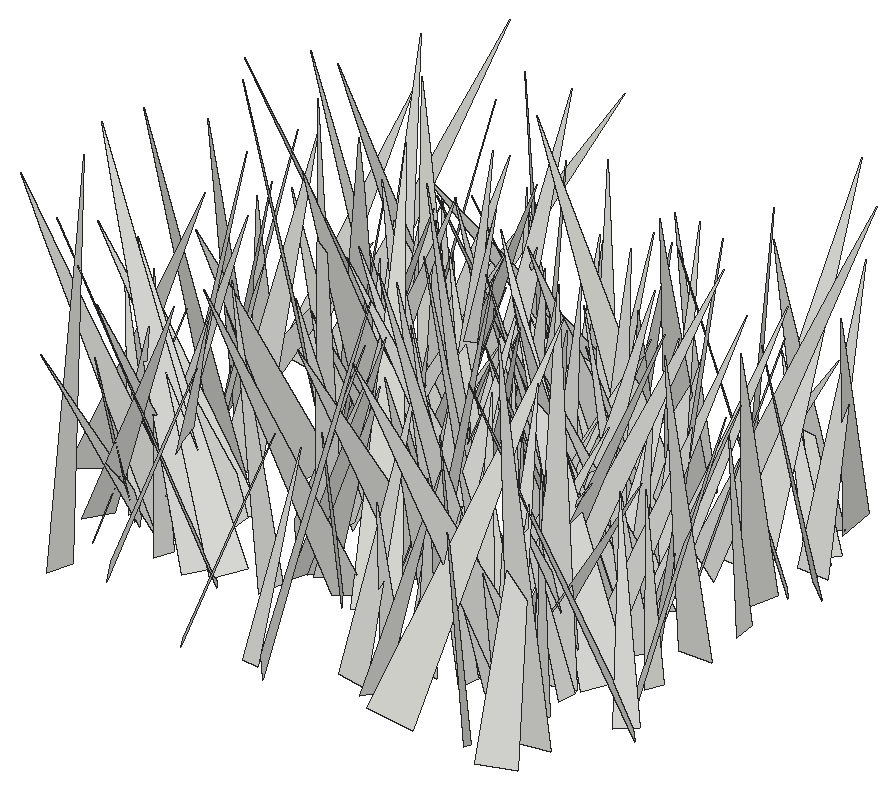
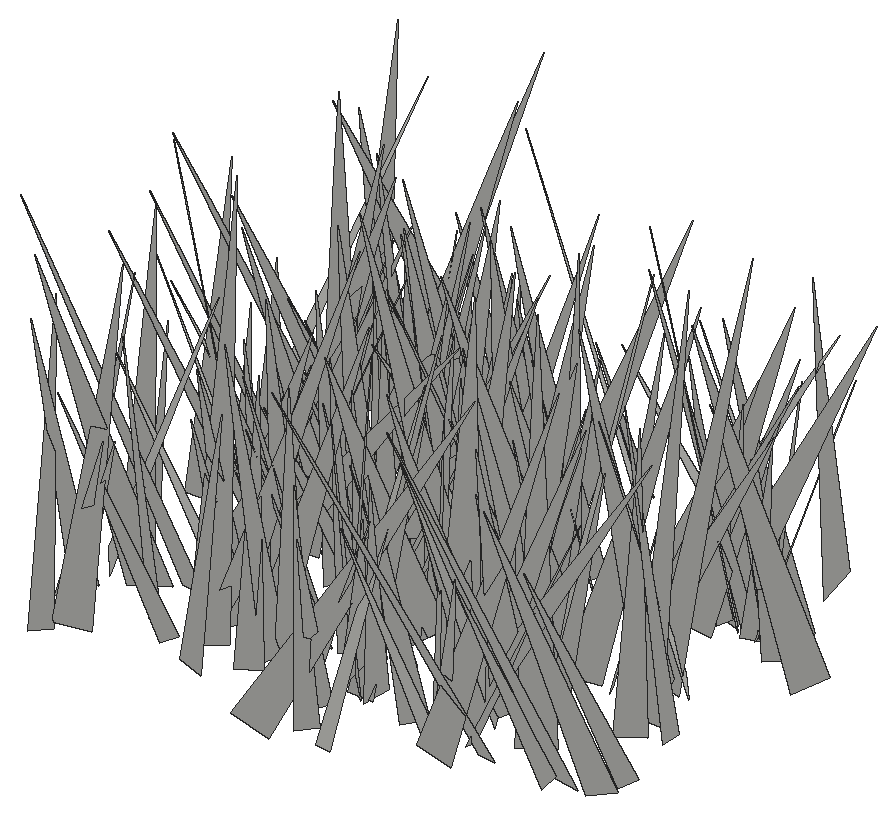
# SketchUp Ruby script. Lengths in inches.
U = 1.inch
M = Sketchup.active_model
def pt(a) = Geom::Point3d.new(a.map { |v| v * U })
def face(e, loops, mat)
  f = e.add_face(loops[0].map { |a| pt(a) })
  loops[1..].each { |l| e.add_face(l.map { |a| pt(a) }).erase! }
  f.material = f.back_material = mat if mat
  f
end
# faces: each face lists its corners as indices into pts; further lists are holes
def faces(e, pts, list, mat = nil) = list.each { |f| face(e, (f[0].is_a?(Array) ? f : [f]).map { |l| l.map { |i| pts[i] } }, mat) }
# xy, xz, yz: faces in a plane at the given z, y or x. An outline is a flat list of corners, or four numbers for a rectangle; further outlines are holes
def ring(l) = l.size == 4 ? [[l[0], l[1]], [l[2], l[1]], [l[2], l[3]], [l[0], l[3]]] : l.each_slice(2).to_a
def flat(e, list, mat, &to3) = list.each { |f| face(e, (f[0].is_a?(Array) ? f : [f]).map { |l| ring(l).map { |u, v| to3.(u, v) } }, mat) }
def xy(e, z, list, mat = nil) = flat(e, list, mat) { |x, y| [x, y, z] }
def xz(e, y, list, mat = nil) = flat(e, list, mat) { |x, z| [x, y, z] }
def yz(e, x, list, mat = nil) = flat(e, list, mat) { |y, z| [x, y, z] }
def lines(e, pts, list) = list.each { |a, b| e.add_line(pt(pts[a]), pt(pts[b])) }
# prism: a flat outline (further loops are holes) pulled along v
def prism(e, loops, v, mat = nil)
  f = face(e, loops, mat); d = Geom::Vector3d.new(v.map { |x| x * U })
  f.pushpull(f.normal.samedirection?(d) ? d.length : -d.length)
end
def box(e, o, s, mat = nil) = prism(e, [[o, [o[0] + s[0], o[1], o[2]], [o[0] + s[0], o[1] + s[1], o[2]], [o[0], o[1] + s[1], o[2]]]], [0, 0, s[2]], mat)
def at(x, y, z, deg = 0) = Geom::Transformation.translation(pt([x, y, z])) * Geom::Transformation.rotation(ORIGIN, Z_AXIS, deg.degrees)
def axes(o, x, y, z) = Geom::Transformation.new([*x, 0, *y, 0, *z, 0, *pt(o).to_a, 1])
def part(name) = M.definitions.add(name)
# library, detail: a bought-in or finely detailed component or shape, given as its bounding box
def library(name, o, s) = part(name).tap { |d| box(d.entities, o, s) }
def detail(e, o, s) = box(e.add_group.entities, o, s)
def put(e, d, t, mat = nil) = e.add_instance(d, t).tap { |i| i.material = mat if mat }
def group(e, t, mat = nil) = e.add_group.tap { |g| g.transformation = t; g.material = mat if mat }.entities
root = M.entities
c1 = part("fur_instance\#9")
p = [[0.8125,0,1.79],[0.67,-0.02,1.48],[0,-0.11,0],[0,0.11,0]]
faces(c1.entities,p,[[0,1,2,3]])
put(root,c1,axes([118.52,285.79,-27.1],[3.43862,2.40363,0.16823],[2.31203,-3.37399,0.94893],[-0.67841,0.6845,4.08669]))
put(root,c1,axes([121.77,286.14,-27.1],[5.53821,4.98185,1.27941],[5.04776,-5.62536,0.05401],[-0.98782,-0.81487,7.449]))
put(root,c1,axes([125.91,287.1,-27.1],[4.66394,-1.20705,1.00362],[-1.36601,-4.67089,0.73033],[-0.77347,0.97077,4.76192]))
put(root,c1,axes([132.45,287.6,-27.1],[0.36283,-7.33481,3.26148],[-7.98321,-0.67122,-0.62142],[-0.83968,3.21222,7.31744]))
put(root,c1,axes([132.47,285.72,-27.1],[-2.78795,6.31949,0.96814],[6.36227,2.84625,-0.25738],[0.62828,-0.78026,6.90234]))
put(root,c1,axes([121.28,286.12,-27.1],[1.03899,3.82207,0.22987],[3.79032,-1.06041,0.49963],[-0.54276,-0.08876,3.92914]))
put(root,c1,axes([131.54,287.22,-27.1],[2.89571,-2.97183,2.13904],[-3.49598,-3.05481,0.48854],[-1.08874,1.90494,4.12046]))
put(root,c1,axes([130.74,286.27,-27.1],[-5.03149,-1.83162,1.20846],[-2.18082,4.50919,-2.24552],[0.24343,2.5384,4.86091]))
put(root,c1,axes([129.28,291.125,-27.1],[-7.73279,0.49202,2.83462],[1.75633,7.24586,3.53356],[2.27869,-3.91518,6.89581]))
put(root,c1,axes([125.46,288.78,-27.1],[2.03457,-2.99845,1.01926],[-3.06758,-2.16697,-0.25148],[-0.78708,0.69471,3.61482]))
put(root,c1,axes([113.4,288.13,-27.1],[4.3525,2.53578,0.43229],[2.57081,-4.2585,-0.90411],[0.08934,-0.99816,4.9555]))
put(root,c1,axes([124.8,287.36,-27.1],[0.44242,5.64748,1.29703],[5.78226,-0.34572,-0.46699],[0.37666,-1.32609,5.6455]))
put(root,c1,axes([127.49,286.0625,-27.1],[-1.94232,7.80928,1.11049],[7.41359,2.19794,-2.48968],[2.69386,-0.41817,7.65238]))
put(root,c1,axes([134.57,290.7,-27.1],[-5.605,-5.08718,0.25266],[-5.09303,5.60246,-0.18084],[0.06544,0.30374,7.56721]))
put(root,c1,axes([111.93,287.25,-27.1],[-7.13651,-0.0123,2.39844],[-0.61978,7.28244,-1.80677],[2.31701,1.91008,6.90402]))
put(root,c1,axes([126.49,289.33,-27.1],[0.16475,-3.83195,1.51207],[-4.1166,-0.0965,0.20397],[0.15418,1.51796,3.83006]))
put(root,c1,axes([126.33,289.23,-27.1],[2.59266,-2.6088,0.97622],[-2.78019,-2.50569,0.68761],[-0.17141,1.18171,3.61316]))
put(root,c1,axes([129.45,289.94,-27.1],[-0.93338,-7.69941,2.7531],[-7.87622,0.10215,-2.38461],[-2.19672,2.90522,7.38009]))
put(root,c1,axes([111.72,291.98,-27.1],[-3.93384,-2.91751,0.42121],[-2.51987,3.69278,2.04402],[1.52955,-1.41982,4.45073]))
put(root,c1,axes([116.91,289.72,-27.1],[-5.49378,-4.48735,0.1731],[-4.21573,5.05933,-2.64174],[-1.54724,2.14821,6.58325]))
put(root,c1,axes([120.97,292.02,-27.1],[0.32689,-6.93131,1.01824],[-6.72809,-0.59471,-1.88835],[-1.95261,0.88881,6.67713]))
put(root,c1,axes([111.3,291.95,-27.1],[-2.16154,-4.08693,0.6496],[-3.73051,2.24163,1.68984],[1.79115,-0.26331,4.30345]))
put(root,c1,axes([110.67,290.95,-27.1],[5.28357,-2.5058,0.04843],[-2.504,-5.27298,0.35108],[0.10676,0.33794,5.83712]))
put(root,c1,axes([120.83,291.77,-27.1],[-2.98653,-2.99705,1.42564],[-2.58075,3.30304,1.53746],[2.08674,-0.20437,3.94181]))
put(root,c1,axes([128.03,289.86,-27.1],[-6.43885,-0.2283,0.73687],[-0.34147,6.39798,-1.00159],[0.69173,1.03328,6.36457]))
put(root,c1,axes([113.85,291.4,-27.1],[-2.36054,6.29762,2.85628],[6.53149,1.03928,3.10644],[-2.27111,-3.55673,5.96508]))
put(root,c1,axes([113.81,292.71,-27.1],[0.77993,-5.26102,0.56712],[-5.12867,-0.89269,-1.22806],[-1.30258,0.36472,5.1748]))
put(root,c1,axes([111.5,289.76,-27.1],[4.04394,2.43918,0.42992],[2.39305,-4.06014,0.52577],[-0.63852,0.23141,4.69325]))
put(root,c1,axes([131.56,289.47,-27.1],[-4.31752,-0.25034,0.73123],[-0.52227,4.00392,-1.71296],[0.56974,1.77322,3.97108]))
put(root,c1,axes([131.33,291.0625,-27.1],[-3.91396,0.19988,0.40503],[0.19284,3.93443,-0.07818],[0.40843,0.05784,3.91828]))
put(root,c1,axes([113.33,291.49,-27.1],[4.73571,-1.08461,0.9225],[-1.0987,-4.82145,-0.02851],[-0.90568,0.17765,4.85824]))
put(root,c1,axes([118.53,290.67,-27.1],[-5.56537,0.35389,1.01892],[0.25962,5.63719,-0.53984],[1.04691,0.48332,5.55042]))
put(root,c1,axes([126.13,289.2,-27.1],[6.62272,2.03005,2.53711],[1.31072,-6.93962,2.13125],[-2.97322,1.46257,6.59085]))
put(root,c1,axes([130.98,293.18,-27.1],[-4.32918,-1.79601,0.73607],[-1.48596,4.22424,1.56749],[1.24875,-1.19977,4.41706]))
put(root,c1,axes([114.15,290.24,-27.1],[-5.02502,0.15502,0.9974],[-0.08895,4.97687,-1.22169],[1.00545,1.21508,4.87671]))
put(root,c1,axes([128.1,290.34,-27.1],[-0.91047,5.0165,1.03079],[5.11456,0.83694,0.44447],[-0.2628,-1.09133,5.07905]))
put(root,c1,axes([116.74,290.58,-27.1],[-3.94655,4.7323,0.06828],[4.56087,3.77904,1.70056],[-1.26405,-1.13963,5.92267]))
put(root,c1,axes([118.87,292.26,-27.1],[6.16535,-1.94029,0.16764],[-1.94054,-6.16752,-0.01601],[-0.16472,0.03505,6.46343]))
put(root,c1,axes([134.27,290.66,-27.1],[-2.51117,3.39602,0.58609],[3.43959,2.51478,0.1658],[0.21361,-0.57041,4.22035]))
put(root,c1,axes([115.94,290.33,-27.1],[-4.22364,6.9226,0.63988],[6.72709,3.88063,2.42031],[-1.75445,-1.78585,7.73974]))
put(root,c1,axes([121.8,295.03,-27.1],[6.11084,-2.63091,1.80363],[-1.49433,-5.80472,-3.40432],[-2.81811,-2.62692,5.71618]))
put(root,c1,axes([110.3,292.7,-27.1],[2.04033,-4.0488,0.48109],[-4.03745,-1.93127,0.8697],[0.56854,0.81522,4.44965]))
put(root,c1,axes([130.5,291.42,-27.1],[1.64686,-6.77743,3.62945],[-7.62252,-1.92308,-0.13234],[-1.0018,3.49096,6.97339]))
put(root,c1,axes([119.25,292.66,-27.1],[4.36325,-2.68491,0.18726],[-2.69098,-4.34538,0.39756],[0.04948,0.43666,5.1077]))
put(root,c1,axes([112.15,291.73,-27.1],[3.4737,5.90005,1.74495],[6.11319,-3.08303,-1.74525],[0.69596,-2.36778,6.62052]))
put(root,c1,axes([128.96,291.46,-27.1],[4.72114,-1.50275,0.05764],[-1.46013,-4.53503,1.361],[0.36002,1.31378,4.76394]))
put(root,c1,axes([113.13,291.31,-27.1],[5.7382,5.20942,1.87337],[5.41352,-5.84467,-0.3291],[-1.15821,-1.50876,7.74318]))
put(root,c1,axes([111.57,291.66,-27.1],[-2.88957,-1.62735,2.00469],[-2.2228,3.09866,-0.68855],[1.31385,1.66334,3.24403]))
put(root,c1,axes([128.09,293.5625,-27.1],[4.34491,0.59069,1.09524],[0.90101,-4.23706,-1.28924],[-0.85828,-1.45776,4.19106]))
put(root,c1,axes([111.79,292.02,-27.1],[-2.18486,3.79279,1.02862],[3.92891,2.13324,0.47945],[0.08359,-1.13179,4.35074]))
put(root,c1,axes([122.86,294.39,-27.1],[2.86729,-4.50295,0.62999],[-4.43501,-2.93396,-0.78577],[-1.00209,0.10064,5.2802]))
put(root,c1,axes([124.1,293.9375,-27.1],[1.75802,-6.33898,1.96931],[-6.51413,-2.03906,-0.74828],[-1.27556,1.67662,6.53555]))
put(root,c1,axes([114.79,293.84,-27.1],[-6.1435,0.43905,0.01492],[0.43419,6.03663,1.1429],[-0.06685,-1.14104,6.05221]))
put(root,c1,axes([125.51,290.25,-27.1],[-5.11664,3.91829,0.85035],[3.38571,4.96082,-2.48663],[2.14782,1.51438,5.94556]))
put(root,c1,axes([127.67,291.82,-27.1],[-6.96753,-1.64469,0.65915],[-1.76863,6.61713,-2.18437],[0.10697,2.27915,6.81763]))
put(root,c1,axes([127.39,293.35,-27.1],[4.14484,0.5886,1.74948],[0.68446,-4.48393,-0.11303],[-1.71425,-0.36717,4.1849]))
put(root,c1,axes([108.24,293.32,-27.1],[6.2285,-2.9564,0.62521],[-3.02175,-6.08711,1.31964],[0.01382,1.46019,6.76705]))
put(root,c1,axes([130.64,294.27,-27.1],[-3.35511,-5.27651,0.83113],[-5.27558,3.11951,-1.49198],[-0.83701,1.48869,6.07225]))
put(root,c1,axes([123.48,295.4375,-27.1],[7.4678,0.08394,0.57516],[0.2355,-7.21321,-2.00499],[-0.53141,-2.01703,7.1941]))
put(root,c1,axes([131.8125,292.59,-27.1],[-7.18183,4.15456,0.03319],[4.14203,7.15453,0.70461],[-0.3242,-0.62648,8.26695]))
put(root,c1,axes([125.59,294.01,-27.1],[2.92691,3.10527,0.26779],[2.82947,-2.4932,-2.01476],[1.3071,-1.55642,3.76168]))
put(root,c1,axes([133.22,293.55,-27.1],[3.01506,-0.72225,2.0256],[-1.00024,-3.559,0.21985],[-1.90373,0.72607,3.09256]))
put(root,c1,axes([114.72,293.96,-27.1],[-4.43376,3.47486,0.22998],[3.34427,4.14468,1.85019],[-0.97128,-1.59146,5.32068]))
put(root,c1,axes([126.64,293.03,-27.1],[0.2906,4.64928,0.9365],[4.41539,0.07727,-1.75374],[1.73123,-0.9775,4.31562]))
put(root,c1,axes([116.67,294.36,-27.1],[3.8282,2.91024,0.83789],[3.01788,-3.55309,-1.44728],[0.25298,-1.65308,4.58585]))
put(root,c1,axes([119.48,292.55,-27.1],[4.39596,-0.31282,2.17467],[-1.10489,-4.51925,1.5834],[-1.89902,1.90528,4.11281]))
put(root,c1,axes([128.0625,292.4,-27.1],[6.72656,-0.08852,1.07497],[-0.40385,-6.50233,1.99163],[-1.00015,2.03024,6.42556]))
put(root,c1,axes([122.38,291.72,-27.1],[-3.14428,7.71271,0.49149],[7.72648,3.12546,0.38342],[-0.17032,-0.59964,8.32018]))
put(root,c1,axes([123.1,291.56,-27.1],[4.98815,3.01806,0.37753],[2.59556,-4.60182,2.49383],[-1.58564,1.9615,5.26983]))
put(root,c1,axes([112.21,296.47,-27.1],[-2.39726,-7.68863,1.50052],[-7.81274,2.46126,0.12966],[0.5725,1.39306,8.05265]))
put(root,c1,axes([128.03,296.89,-27.1],[0.49777,-7.47829,0.86543],[-7.52286,-0.52678,-0.22508],[-0.28353,0.84808,7.49146]))
put(root,c1,axes([126.61,293.875,-27.1],[-4.17339,1.81444,1.20525],[1.74242,4.34394,-0.50613],[1.30721,0.0026,4.52253]))
put(root,c1,axes([125.91,293.68,-27.1],[-7.81157,-0.92448,1.21309],[-1.13809,7.74743,-1.42443],[1.01538,1.5715,7.73604]))
put(root,c1,axes([117.86,296.0625,-27.1],[-4.50462,1.14541,2.32905],[1.86637,4.67145,1.31236],[1.80364,-1.97324,4.45884]))
put(root,c1,axes([133.42,292.21,-27.1],[3.56764,3.88458,0.34534],[3.52617,-3.41301,1.96335],[-1.66594,1.09483,4.89523]))
put(root,c1,axes([124.53,296.16,-27.1],[-6.85321,0.30824,0.48855],[0.41589,6.6696,1.62593],[0.40091,-1.64973,6.66467]))
put(root,c1,axes([114.72,297.91,-27.1],[4.75153,-4.99406,0.9078],[-4.47168,-4.70683,-2.48828],[-2.40183,-1.11663,6.42854]))
put(root,c1,axes([126.08,293.71,-27.1],[-6.2227,2.39174,0.32304],[2.36421,6.22042,-0.51348],[0.48507,0.36431,6.64671]))
put(root,c1,axes([128.19,292.97,-27.1],[3.14457,7.68443,0.45621],[7.56933,-2.99688,-1.69436],[1.40136,-1.05601,8.12822]))
put(root,c1,axes([118.64,293.78,-27.1],[-8.04005,-0.21045,2.18635],[-0.63833,8.16213,-1.56173],[2.10165,1.67397,7.88972]))
put(root,c1,axes([133,296.08,-27.1],[0.27233,-6.25887,1.87066],[-6.53155,-0.29195,-0.02597],[-0.1084,1.8677,6.26474]))
put(root,c1,axes([122.85,296.15,-27.1],[-6.22259,1.31552,1.1088],[1.51746,6.15727,1.21077],[0.81078,-1.42761,6.24382]))
put(root,c1,axes([129.53,295.08,-27.1],[-6.43064,-2.17008,0.24743],[-2.17262,6.27662,-1.4168],[-0.22404,1.42068,6.6374]))
put(root,c1,axes([124.13,292.73,-27.1],[-7.73799,2.57835,1.8542],[1.9672,7.72518,-2.53263],[2.4932,1.90688,7.75308]))
put(root,c1,axes([122.16,296.6875,-27.1],[1.97582,-3.11414,0.08334],[-3.10691,-1.9626,0.3224],[0.22782,0.24287,3.67393]))
put(root,c1,axes([123.75,297.17,-27.1],[-4.70083,-1.74871,0.0814],[-1.70109,4.61801,0.97093],[0.41342,-0.88228,4.92068]))
put(root,c1,axes([122.21,294.58,-27.1],[6.62959,-1.41825,2.66639],[-1.99694,-6.88369,1.30369],[-2.26567,1.91728,6.65307]))
put(root,c1,axes([129.83,296.74,-27.1],[-3.46593,0.7925,0.89611],[1.04093,3.35143,1.06213],[0.58952,-1.25841,3.39303]))
put(root,c1,axes([119.54,296.45,-27.1],[4.26328,-1.39926,0.74192],[-1.39292,-4.32659,-0.15583],[-0.75375,0.08115,4.48433]))
put(root,c1,axes([126.78,296.35,-27.1],[2.27684,-3.73592,1.683],[-3.94498,-2.51908,-0.25488],[-1.10756,1.29258,4.36763]))
put(root,c1,axes([130.36,293.97,-27.1],[2.81698,6.47491,0.35167],[6.46114,-2.77024,-0.75032],[0.54938,-0.62035,7.02117]))
put(root,c1,axes([116.74,296.75,-27.1],[-6.42891,-4.93695,1.78859],[-5.18873,6.40682,-0.96596],[0.80598,1.86616,8.04806]))
put(root,c1,axes([113.43,297.87,-27.1],[-3.15969,-2.10838,0.70871],[-1.88389,3.19122,1.09464],[1.18257,-0.54957,3.6374]))
put(root,c1,axes([124.48,297.24,-27.1],[4.31409,-4.88001,1.43702],[-5.06352,-4.30068,0.59646],[-0.49016,1.47666,6.48614]))
put(root,c1,axes([124.73,296.18,-27.1],[0.74077,3.76285,1.03817],[3.63302,-0.27816,-1.5841],[1.42759,-1.24465,3.49262]))
put(root,c1,axes([132.1,294.93,-27.1],[5.36611,5.59511,2.05394],[5.5109,-5.71038,1.15783],[-2.27022,-0.63666,7.66549]))
put(root,c1,axes([130.46,296.2,-27.1],[4.29759,3.17988,0.45483],[3.21134,-4.23507,-0.73441],[0.07624,-0.86047,5.29543]))
put(root,c1,axes([130.17,297.79,-27.1],[0.21984,-5.04241,1.33274],[-4.72838,-0.75562,-2.0789],[-2.20101,1.11963,4.59917]))
put(root,c1,axes([127.36,295.63,-27.1],[0.34617,6.42334,1.62872],[6.51894,-0.03728,-1.2385],[1.18972,-1.66468,6.31231]))
put(root,c1,axes([120.54,297.25,-27.1],[-3.35147,5.54659,2.9979],[6.27053,3.28643,0.92965],[0.65767,-3.06906,6.41348]))
put(root,c1,axes([111.07,298.81,-27.1],[-1.7083,-7.51191,1.45388],[-7.48357,1.95063,1.28533],[1.59333,1.10775,7.59572]))
put(root,c1,axes([121.02,294.93,-27.1],[4.46685,2.95329,0.59597],[2.75098,-4.43263,1.34675],[-1.2285,0.81223,5.18275]))
put(root,c1,axes([131.4,295,-27.1],[0.1109,6.16383,0.84068],[5.38265,-0.51661,3.07768],[-3.11876,-0.67243,5.34163]))
put(root,c1,axes([116.37,296.59,-27.1],[6.24865,-3.61776,1.18124],[-3.80474,-5.99015,1.78079],[-0.08657,2.13519,6.99733]))
put(root,c1,axes([117.35,296.39,-27.1],[4.17015,5.48726,0.52169],[5.30168,-3.81404,-2.26221],[1.50809,-1.76505,6.51019]))
put(root,c1,axes([112.43,296.625,-27.1],[-0.87926,6.56228,2.62812],[6.83144,1.46959,-1.38397],[1.81713,-2.34956,6.47466]))
put(root,c1,axes([117.02,299.56,-27.1],[-4.18199,-2.55213,0.91155],[-1.98836,4.02848,2.15666],[1.84139,-1.44616,4.39901]))
put(root,c1,axes([115.78,301,-27.1],[5.60712,-6.07402,0.33398],[-5.83929,-5.5015,-2.02021],[-1.70529,-1.13347,8.01575]))
put(root,c1,axes([118.68,297.21,-27.1],[2.58495,3.56171,0.23056],[3.43761,-2.40789,-1.34382],[0.96012,-0.96809,4.1907]))
put(root,c1,axes([129.06,297.71,-27.1],[0.06663,3.86387,1.64805],[4.18879,0.06273,-0.31643],[0.31563,-1.6482,3.85147]))
put(root,c1,axes([120.68,298.73,-27.1],[5.22033,-0.21574,2.13038],[0.1303,-5.5713,-0.88347],[-2.13731,-0.86658,5.14955]))
put(root,c1,axes([111.57,295.97,-27.1],[4.49985,4.45709,1.03745],[4.28289,-4.6143,1.2473],[-1.61209,0.1822,6.20956]))
put(root,c1,axes([125.49,297.71,-27.1],[-4.36102,2.95909,2.58691],[3.11538,4.95832,-0.41976],[2.39639,-1.06094,5.25343]))
put(root,c1,axes([130.69,296.01,-27.1],[1.99959,6.47326,0.24716],[6.43471,-1.95494,-0.85747],[0.74746,-0.48749,6.72058]))
put(root,c1,axes([133.22,298.52,-27.1],[3.59976,0.06174,1.80471],[0.19659,-4.01441,-0.2548],[-1.79504,-0.31584,3.59126]))
put(root,c1,axes([109.68,299.28,-27.1],[5.83398,1.13984,1.03884],[1.35175,-5.73614,-1.2974],[-0.74243,-1.48703,5.80098]))
put(root,c1,axes([128.625,298,-27.1],[-5.00631,-5.98003,0.73957],[-5.22244,3.82659,-4.41068],[-3.00563,3.31169,6.43193]))
put(root,c1,axes([118.12,299.5,-27.1],[8.10386,-2.02713,0.06413],[-2.02706,-8.10412,-0.01624],[-0.06615,-0.00019,8.35354]))
put(root,c1,axes([123.91,298.3,-27.1],[3.88682,0.49651,1.01606],[0.42112,-4.01087,0.34905],[-1.04955,0.22945,3.90283]))
put(root,c1,axes([110.85,300.03,-27.1],[3.52243,-4.25283,0.7835],[-4.27225,-3.57882,-0.21878],[-0.66956,0.46198,5.5178]))
put(root,c1,axes([128.56,296.8,-27.1],[-0.5351,4.97369,0.08314],[4.96853,0.53845,-0.2337],[0.24128,-0.05757,4.99693]))
put(root,c1,axes([132.36,300.48,-27.1],[5.38586,-3.00561,1.16634],[-2.8404,-5.49795,-1.05176],[-1.52519,-0.37466,6.07741]))
put(root,c1,axes([123.78,298.3,-27.1],[-0.24087,4.17753,0.95098],[3.88217,0.61574,-1.72155],[1.81241,-0.76371,3.81393]))
put(root,c1,axes([114.31,300.125,-27.1],[6.51578,-0.90085,0.09034],[-0.89347,-6.50413,-0.41604],[-0.1463,-0.39981,6.56459]))
put(root,c1,axes([128.46,300.25,-27.1],[-4.34148,-1.68145,0.56308],[-1.64517,4.37512,0.38015],[0.66161,-0.1544,4.64018]))
put(root,c1,axes([115.09,298.58,-27.1],[4.32331,2.64676,1.47041],[2.57631,-4.56233,0.63737],[-1.59061,-0.19566,5.02892]))
put(root,c1,axes([122.63,300.2,-27.1],[-6.25427,-0.78477,1.30734],[-0.71032,6.38344,0.43371],[1.34924,-0.27711,6.28838]))
put(root,c1,axes([122.125,301.38,-27.1],[0.90872,-5.0896,0.45336],[-4.90772,-0.74115,1.51668],[1.42262,0.69427,4.94262]))
put(root,c1,axes([116.06,299.3,-27.1],[-2.49672,2.92464,0.96124],[2.97957,2.60694,-0.1927],[0.77439,-0.6012,3.84057]))
put(root,c1,axes([117.77,300.77,-27.1],[1.5026,-5.2869,1.47769],[-5.48951,-1.44343,0.41772],[0.01326,1.53554,5.48039]))
put(root,c1,axes([126.15,299.76,-27.1],[-1.18817,5.57554,2.26119],[5.96275,1.39894,-0.31626],[0.80332,-2.13721,5.69196]))
put(root,c1,axes([113.52,301,-27.1],[-4.62696,1.13691,1.70574],[1.48296,4.76376,0.84751],[1.41525,-1.27471,4.68861]))
put(root,c1,axes([118.45,300.07,-27.1],[5.58768,-4.04107,3.86555],[-4.58295,-6.44048,-0.10822],[-3.20457,2.16447,6.89498]))
put(root,c1,axes([112.9,302.69,-27.1],[1.80193,-7.44469,0.50754],[-7.36471,-1.69029,1.35351],[1.20089,0.80465,7.53912]))
put(root,c1,axes([116.81,298.84,-27.1],[-4.46885,1.59045,1.08144],[1.18804,4.43404,-1.61169],[1.51249,1.21632,4.46123]))
put(root,c1,axes([130.43,298.92,-27.1],[4.1336,3.03674,0.5342],[2.87698,-4.11997,1.15876],[-1.10914,0.6308,4.99657]))
put(root,c1,axes([121.27,301.39,-27.1],[3.01124,-3.84874,1.35887],[-4.04465,-3.04041,0.35153],[-0.54781,1.29229,4.87409]))
put(root,c1,axes([133.38,302.35,-27.1],[-3.17607,-4.40082,1.193],[-4.40846,3.33508,0.56622],[1.16445,0.62283,5.3976]))
put(root,c1,axes([124.6,303.1875,-27.1],[2.95346,-5.37759,1.21149],[-5.08452,-3.18852,-1.75785],[-2.12927,0.1548,5.87804]))
put(root,c1,axes([126.3,304.08,-27.1],[7.64117,-3.1953,0.94942],[-2.87226,-7.51641,-2.18001],[-1.69158,-1.67105,7.9903]))
put(root,c1,axes([119.57,300.94,-27.1],[3.16954,2.48643,0.53995],[2.54162,-3.13416,-0.48689],[-0.1185,-0.71733,3.99891]))
put(root,c1,axes([132.68,301.58,-27.1],[-5.08452,-4.09315,0.88657],[-4.17476,4.84247,-1.58557],[-0.33349,1.78573,6.33184]))
put(root,c1,axes([125.1875,299.67,-27.1],[1.99951,5.4557,0.6063],[5.41529,-2.06607,0.73224],[-0.89823,-0.31139,5.76424]))
put(root,c1,axes([126.85,302.43,-27.1],[-8.04315,1.60644,1.39343],[1.83623,7.99603,1.38066],[1.07265,-1.64234,8.08496]))
put(root,c1,axes([116.71,303.48,-27.1],[-2.8265,-4.26887,1.57231],[-3.66111,3.23328,2.19698],[2.70032,-0.08465,4.62446]))
put(root,c1,axes([119.9375,303.62,-27.1],[-0.22883,-5.12281,0.23524],[-5.12454,0.23734,0.18366],[0.19416,0.22665,5.12463]))
put(root,c1,axes([123.05,301.53,-27.1],[2.48404,3.35431,0.63876],[3.34518,-2.23213,-1.28736],[0.685,-1.26336,3.97047]))
put(root,c1,axes([116.55,301.2,-27.1],[-3.06653,-6.21678,2.70439],[-6.51984,1.89062,-3.04678],[-1.85842,3.62531,6.22648]))
put(root,c1,axes([116.33,300.99,-27.1],[-3.15581,4.82371,2.67558],[4.59437,4.00448,-1.80054],[3.05265,-1.04019,5.47589]))
put(root,c1,axes([128.9,299.4375,-27.1],[0.42359,6.38348,0.10104],[6.1795,-0.43539,1.60081],[-1.60398,0.00839,6.194]))
put(root,c1,axes([120.72,299.03,-27.1],[-6.29891,4.40553,1.36932],[3.82289,6.28157,-2.62437],[2.58248,1.44677,7.22479]))
put(root,c1,axes([114.84,303.875,-27.1],[-4.29176,-1.39668,0.34406],[-1.22552,4.11722,1.42648],[0.75311,-1.25938,4.28195]))
put(root,c1,axes([116.16,302.47,-27.1],[-4.67528,-5.85921,0.505],[-5.43274,4.05599,-3.23694],[-2.25181,2.37953,6.76097]))
put(root,c1,axes([126.36,302.19,-27.1],[-1.839,3.01934,1.93742],[3.07994,2.44517,-0.88715],[1.83955,-1.07548,3.42218]))
put(root,c1,axes([108.84,302.66,-27.1],[1.93678,-3.59499,0.72466],[-3.24209,-1.29543,2.2385],[1.71404,1.61186,3.41529]))
put(root,c1,axes([129.13,301.34,-27.1],[3.76818,7.24013,0.96766],[7.17608,-3.46602,-2.01138],[1.36373,-1.76699,7.91031]))
put(root,c1,axes([124.14,304.53,-27.1],[1.58205,-4.94043,0.08132],[-4.90313,-1.55912,0.66773],[0.6114,0.28046,5.1444]))
put(root,c1,axes([123.96,303.33,-27.1],[5.74343,-0.59024,1.12729],[-0.57342,-5.85294,-0.14303],[-1.13593,-0.02976,5.77191]))
put(root,c1,axes([117.33,303.84,-27.1],[2.31038,-4.41979,0.71264],[-4.3801,-2.06578,1.38834],[0.92579,1.25629,4.79008]))
put(root,c1,axes([115.32,305.3,-27.1],[-0.75565,-7.24529,1.23648],[-7.25287,0.53359,-1.30585],[-1.19119,1.34729,7.16659]))
put(root,c1,axes([115.15,301.17,-27.1],[-6.13848,3.83375,0.83292],[3.60337,6.1212,-1.61832],[1.55148,0.95163,7.05405]))
put(root,c1,axes([121.12,302.82,-27.1],[-6.29577,-3.22015,2.48262],[-3.79064,6.30377,-1.43636],[1.47099,2.46225,6.92409]))
put(root,c1,axes([115.46,301.58,-27.1],[5.32876,3.34285,1.26399],[2.90072,-5.37113,1.97605],[-2.08763,1.0697,5.97207]))
put(root,c1,axes([123.51,302.97,-27.1],[-0.65155,5.99766,1.58433],[6.18323,0.49957,0.65163],[-0.49968,-1.63861,5.99765]))
put(root,c1,axes([120.32,303.33,-27.1],[3.4021,4.35261,1.87369],[4.47593,-3.70904,0.48912],[-1.55627,-1.15238,5.50275]))
put(root,c1,axes([118.68,307.25,-27.1],[-3.43446,-5.67079,0.15135],[-5.3482,3.29577,2.1239],[1.89143,-0.97791,6.28032]))
put(root,c1,axes([119.51,303.27,-27.1],[-4.59387,1.36569,1.34916],[1.20913,4.77619,-0.71765],[1.49109,0.33451,4.73854]))
put(root,c1,axes([132.42,303.65,-27.1],[-3.36159,2.04077,0.19725],[2.04893,3.35754,0.1809],[0.07444,-0.25709,3.9284]))
put(root,c1,axes([121.63,307.625,-27.1],[2.28844,-6.77562,0.58153],[-5.77223,-2.2597,-3.61376],[-3.59563,-0.68473,6.17144]))
put(root,c1,axes([129.58,303.02,-27.1],[-5.36603,-1.88935,2.74168],[-2.67241,5.54565,-1.40882],[1.98613,2.35731,5.51173]))
put(root,c1,axes([130.5,302.0625,-27.1],[-1.86477,7.56726,1.18834],[7.49142,2.05683,-1.34204],[1.5982,-0.81177,7.67722]))
put(root,c1,axes([130.8125,305.99,-27.1],[2.01145,-6.31603,1.30369],[-6.40118,-2.12156,-0.40211],[-0.78536,1.11557,6.61638]))
put(root,c1,axes([132.5,303.21,-27.1],[-0.07417,5.83715,1.21265],[5.95855,0.11247,-0.17697],[0.19614,-1.2097,5.83493]))
put(root,c1,axes([120.58,303.16,-27.1],[-3.8761,2.85036,0.12124],[2.83481,3.87102,-0.37744],[0.32105,0.23257,4.79648]))
put(root,c1,axes([127.61,304.59,-27.1],[1.13497,4.33314,1.68645],[4.04549,-0.06445,-2.557],[2.29221,-2.03177,3.67778]))
put(root,c1,axes([121.97,303.65,-27.1],[-4.83845,-0.36416,0.05457],[-0.36621,4.6838,-1.21411],[-0.03844,1.21473,4.69778]))
put(root,c1,axes([116.12,303.94,-27.1],[0.1057,3.9764,0.92499],[3.9126,-0.36287,1.11284],[-1.16573,-0.85739,3.81897]))
put(root,c1,axes([109.125,303.75,-27.1],[-0.64371,5.67181,1.6895],[5.48083,1.21245,-1.9821],[2.23257,-1.34117,5.35305]))
put(root,c1,axes([132.23,304.49,-27.1],[-2.23276,3.13779,0.67741],[3.20125,2.1153,0.75324],[-0.23799,-0.9847,3.77672]))
put(root,c1,axes([131.5,306.85,-27.1],[5.7747,-1.11479,0.95698],[-0.77258,-5.60537,-1.86777],[-1.24967,-1.68603,5.57685]))
put(root,c1,axes([111.04,304.28,-27.1],[4.1398,0.29454,0.02134],[0.28882,-4.10074,0.57065],[-0.06159,0.56772,4.11084]))
put(root,c1,axes([116.41,304.24,-27.1],[4.19181,1.99584,0.5753],[1.88629,-4.2003,0.82769],[-0.86965,0.50967,4.56832]))
put(root,c1,axes([125.84,305.64,-27.1],[-1.40726,-4.75955,2.034],[-5.17479,1.24906,-0.65748],[-0.10975,2.13481,4.91949]))
put(root,c1,axes([113.78,304.29,-27.1],[4.07618,6.66518,0.05677],[6.29765,-3.82934,-2.59208],[2.18344,-1.39809,7.37028]))
put(root,c1,axes([119.95,306.56,-27.1],[3.72524,-2.31212,0.81738],[-2.32656,-3.80205,-0.15146],[-0.77532,0.29988,4.38182]))
put(root,c1,axes([120.54,305.05,-27.1],[-2.95191,2.4359,0.97471],[2.3622,3.10602,-0.60836],[1.1418,-0.12828,3.77853]))
put(root,c1,axes([110.49,304.02,-27.1],[3.27574,7.01328,0.4286],[6.91428,-3.13335,-1.57325],[1.25002,-1.04703,7.57902]))
